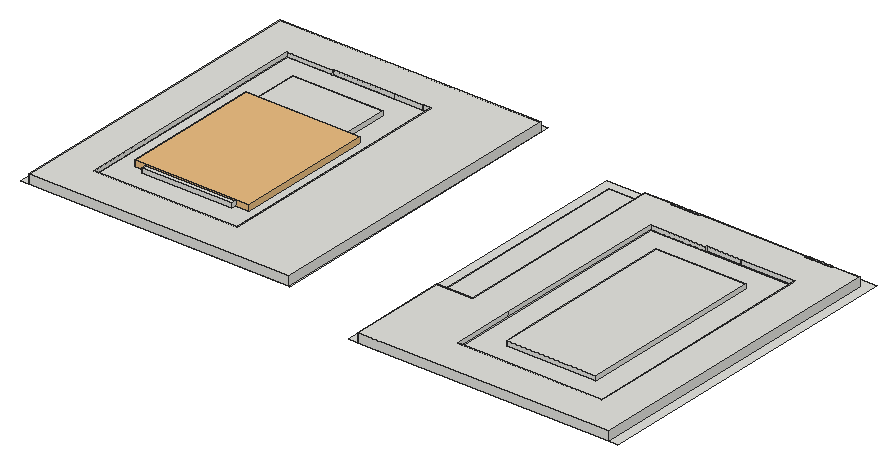
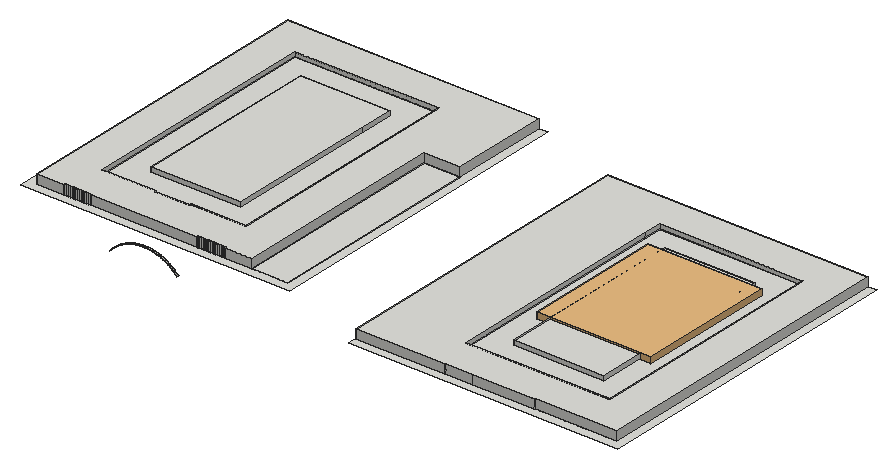
# SketchUp Ruby script. Lengths in inches.
U = 1.inch
M = Sketchup.active_model
def pt(a) = Geom::Point3d.new(a.map { |v| v * U })
def face(e, loops, mat)
  f = e.add_face(loops[0].map { |a| pt(a) })
  loops[1..].each { |l| e.add_face(l.map { |a| pt(a) }).erase! }
  f.material = f.back_material = mat if mat
  f
end
# faces: each face lists its corners as indices into pts; further lists are holes
def faces(e, pts, list, mat = nil) = list.each { |f| face(e, (f[0].is_a?(Array) ? f : [f]).map { |l| l.map { |i| pts[i] } }, mat) }
# xy, xz, yz: faces in a plane at the given z, y or x. An outline is a flat list of corners, or four numbers for a rectangle; further outlines are holes
def ring(l) = l.size == 4 ? [[l[0], l[1]], [l[2], l[1]], [l[2], l[3]], [l[0], l[3]]] : l.each_slice(2).to_a
def flat(e, list, mat, &to3) = list.each { |f| face(e, (f[0].is_a?(Array) ? f : [f]).map { |l| ring(l).map { |u, v| to3.(u, v) } }, mat) }
def xy(e, z, list, mat = nil) = flat(e, list, mat) { |x, y| [x, y, z] }
def xz(e, y, list, mat = nil) = flat(e, list, mat) { |x, z| [x, y, z] }
def yz(e, x, list, mat = nil) = flat(e, list, mat) { |y, z| [x, y, z] }
def lines(e, pts, list) = list.each { |a, b| e.add_line(pt(pts[a]), pt(pts[b])) }
# prism: a flat outline (further loops are holes) pulled along v
def prism(e, loops, v, mat = nil)
  f = face(e, loops, mat); d = Geom::Vector3d.new(v.map { |x| x * U })
  f.pushpull(f.normal.samedirection?(d) ? d.length : -d.length)
end
def box(e, o, s, mat = nil) = prism(e, [[o, [o[0] + s[0], o[1], o[2]], [o[0] + s[0], o[1] + s[1], o[2]], [o[0], o[1] + s[1], o[2]]]], [0, 0, s[2]], mat)
def at(x, y, z, deg = 0) = Geom::Transformation.translation(pt([x, y, z])) * Geom::Transformation.rotation(ORIGIN, Z_AXIS, deg.degrees)
def axes(o, x, y, z) = Geom::Transformation.new([*x, 0, *y, 0, *z, 0, *pt(o).to_a, 1])
def part(name) = M.definitions.add(name)
# library, detail: a bought-in or finely detailed component or shape, given as its bounding box
def library(name, o, s) = part(name).tap { |d| box(d.entities, o, s) }
def detail(e, o, s) = box(e.add_group.entities, o, s)
def put(e, d, t, mat = nil) = e.add_instance(d, t).tap { |i| i.material = mat if mat }
def group(e, t, mat = nil) = e.add_group.tap { |g| g.transformation = t; g.material = mat if mat }.entities
root = M.entities
M.materials.add("[Color M00]").color = [255, 255, 255]
c1 = library("ceiling fan",[0,0,0],[76.25,93.13,30.02])
c2 = part("Component\#2")
xy(c2.entities,0,[[3.27,0,4.25,0.01,5.2,0.27,6.04,0.77,6.72,1.47,7.2,2.33,7.45,3.27,7.44,4.25,7.17,5.2,6.67,6.04,5.97,6.72,5.12,7.2,4.17,7.45,3.19,7.44,2.25,7.17,1.41,6.67,0.72,5.97,0.24,5.12,0,4.17,0.01,3.19,0.27,2.25,0.77,1.41,1.47,0.72,2.33,0.24]],"[Color M00]")
xy(root,117.8,[[268.823,66.2,269.003,89.8],[268.823,90.2,269.003,113.8],[268.823,114.2,269.003,137.8],[268.823,138.2,269.003,161.8],[268.823,162.2,269.003,185.8],
  [268.823,186.2,269.003,209.8]])
xy(root,118,[[245.003,66,268.823,210],[268.823,66,269.003,210]])
xy(root,118.8,[[150,61.77,150.18,89.203],[150,89.603,150.18,118.037],[150,118.437,150.18,146.87],[150,147.27,150.18,175.703],[150,176.103,150.18,204.537],
  [150,204.937,150.18,233.37]])
xy(root,119,[[150,61.57,150.18,233.57]])
xy(root,120,[[239.003,0,245.003,0,245.003,210,413.003,210,413.003,0,419.003,0,419.003,216,239.003,216],[[245.003,0,245.003,66,269.003,66,269.003,210,287.003,210,287.003,209,288.003,209,288.003,210,288.203,210,288.203,209,289.203,209,289.203,210,289.403,210,289.403,209,290.403,209,290.403,210,290.603,210,290.603,209,291.603,209,291.603,210,291.803,210,291.803,209,292.803,209,292.803,210,293.003,210,293.003,209,294.003,209,294.003,210,294.203,210,294.203,209,295.203,209,295.203,210,295.403,210,295.403,209,296.403,209,296.403,210,296.603,210,296.603,209,297.603,209,297.603,210,297.803,210,297.803,209,298.803,209,298.803,210,299.003,210,299.003,209,300.003,209,300.003,210,300.203,210,300.203,209,301.203,209,301.203,210,301.403,210,301.403,209,302.403,209,302.403,210,302.603,210,302.603,209,303.603,209,303.603,210,303.803,210,303.803,209,304.803,209,304.803,210,305.003,210,305.003,209,306.003,209,306.003,210,377.003,210,377.003,209,378.003,209,378.003,210,378.203,210,378.203,209,379.203,209,379.203,210,379.403,210,379.403,209,380.403,209,380.403,210,380.603,210,380.603,209,381.603,209,381.603,210,381.803,210,381.803,209,382.803,209,382.803,210,383.003,210,383.003,209,384.003,209,384.003,210,384.203,210,384.203,209,385.203,209,385.203,210,385.403,210,385.403,209,386.403,209,386.403,210,386.603,210,386.603,209,387.603,209,387.603,210,387.803,210,387.803,209,388.803,209,388.803,210,389.003,210,389.003,209,390.166,209,390.166,210,390.366,210,390.366,209,391.366,209,391.366,210,391.566,210,391.566,209,392.728,209,392.728,210,392.928,210,392.928,209,393.928,209,393.928,210,394.128,210,394.128,209,395.003,209,395.003,210,413.003,210,413.003,0],[293.003,24,389.003,185],[313.331,193.1875,314.608,193.365,315.795,193.867,316.812,194.659,317.589,195.687,318.074,196.881,318.233,198.16,318.056,199.437,317.554,200.624,316.762,201.641,315.734,202.419,314.539,202.903,313.26,203.0625,311.984,202.885,310.796,202.383,309.779,201.591,309.002,200.563,308.517,199.369,308.358,198.09,308.536,196.813,309.038,195.626,309.83,194.609,310.858,193.831,312.052,193.347],[357.331,193.1875,358.608,193.365,359.795,193.867,360.812,194.659,361.589,195.687,362.074,196.881,362.233,198.16,362.056,199.437,361.554,200.624,360.762,201.641,359.734,202.419,358.539,202.903,357.26,203.0625,355.984,202.885,354.796,202.383,353.779,201.591,353.002,200.563,352.517,199.369,352.358,198.09,352.536,196.813,353.038,195.626,353.83,194.609,354.858,193.831,356.052,193.347],[281.456,7.0625,282.733,7.24,283.92,7.742,284.937,8.534,285.714,9.562,286.199,10.756,286.358,12.035,286.181,13.312,285.679,14.499,284.887,15.516,283.859,16.294,282.664,16.778,281.385,16.9375,280.109,16.76,278.921,16.258,277.904,15.466,277.127,14.438,276.642,13.244,276.483,11.965,276.661,10.688,277.163,9.501,277.955,8.484,278.983,7.706,280.177,7.222],[399.769,7.0625,401.045,7.24,402.233,7.742,403.25,8.534,404.027,9.562,404.512,10.756,404.671,12.035,404.493,13.312,403.991,14.499,403.199,15.516,402.171,16.294,400.977,16.778,399.698,16.9375,398.421,16.76,397.234,16.258,396.217,15.466,395.44,14.438,394.955,13.244,394.796,11.965,394.973,10.688,395.475,9.501,396.267,8.484,397.295,7.706,398.49,7.222],[313.331,7.0625,314.608,7.24,315.795,7.742,316.812,8.534,317.589,9.562,318.074,10.756,318.233,12.035,318.056,13.312,317.554,14.499,316.762,15.516,315.734,16.294,314.539,16.778,313.26,16.9375,311.984,16.76,310.796,16.258,309.779,15.466,309.002,14.438,308.517,13.244,308.358,11.965,308.536,10.688,309.038,9.501,309.83,8.484,310.858,7.706,312.052,7.222],[357.331,7.0625,358.608,7.24,359.795,7.742,360.812,8.534,361.589,9.562,362.074,10.756,362.233,12.035,362.056,13.312,361.554,14.499,360.762,15.516,359.734,16.294,358.539,16.778,357.26,16.9375,355.984,16.76,354.796,16.258,353.779,15.466,353.002,14.438,352.517,13.244,352.358,11.965,352.536,10.688,353.038,9.501,353.83,8.484,354.858,7.706,356.052,7.222],[281.456,89.875,282.733,90.053,283.92,90.554,284.937,91.346,285.714,92.374,286.199,93.569,286.358,94.848,286.181,96.125,285.679,97.312,284.887,98.329,283.859,99.106,282.664,99.591,281.385,99.75,280.109,99.572,278.921,99.071,277.904,98.279,277.127,97.251,276.642,96.056,276.483,94.777,276.661,93.5,277.163,92.313,277.955,91.296,278.983,90.519,280.177,90.034],[399.769,89.875,401.045,90.053,402.233,90.554,403.25,91.346,404.027,92.374,404.512,93.569,404.671,94.848,404.493,96.125,403.991,97.312,403.199,98.329,402.171,99.106,400.977,99.591,399.698,99.75,398.421,99.572,397.234,99.071,396.217,98.279,395.44,97.251,394.955,96.056,394.796,94.777,394.973,93.5,395.475,92.313,396.267,91.296,397.295,90.519,398.49,90.034],[399.769,53.6875,401.045,53.865,402.233,54.367,403.25,55.159,404.027,56.187,404.512,57.381,404.671,58.66,404.493,59.937,403.991,61.124,403.199,62.141,402.171,62.919,400.977,63.403,399.698,63.5625,398.421,63.385,397.234,62.883,396.217,62.091,395.44,61.063,394.955,59.869,394.796,58.59,394.973,57.313,395.475,56.126,396.267,55.109,397.295,54.331,398.49,53.847],[281.456,53.6875,282.733,53.865,283.92,54.367,284.937,55.159,285.714,56.187,286.199,57.381,286.358,58.66,286.181,59.937,285.679,61.124,284.887,62.141,283.859,62.919,282.664,63.403,281.385,63.5625,280.109,63.385,278.921,62.883,277.904,62.091,277.127,61.063,276.642,59.869,276.483,58.59,276.661,57.313,277.163,56.126,277.955,55.109,278.983,54.331,280.177,53.847],[281.456,137.125,282.733,137.303,283.92,137.804,284.937,138.596,285.714,139.624,286.199,140.819,286.358,142.098,286.181,143.375,285.679,144.562,284.887,145.579,283.859,146.356,282.664,146.841,281.385,147,280.109,146.822,278.921,146.321,277.904,145.529,277.127,144.501,276.642,143.306,276.483,142.027,276.661,140.75,277.163,139.563,277.955,138.546,278.983,137.769,280.177,137.284],[399.769,137.125,401.045,137.303,402.233,137.804,403.25,138.596,404.027,139.624,404.512,140.819,404.671,142.098,404.493,143.375,403.991,144.562,403.199,145.579,402.171,146.356,400.977,146.841,399.698,147,398.421,146.822,397.234,146.321,396.217,145.529,395.44,144.501,394.955,143.306,394.796,142.027,394.973,140.75,395.475,139.563,396.267,138.546,397.295,137.769,398.49,137.284],[281.456,190.125,282.733,190.303,283.92,190.804,284.937,191.596,285.714,192.624,286.199,193.819,286.358,195.098,286.181,196.375,285.679,197.562,284.887,198.579,283.859,199.356,282.664,199.841,281.385,200,280.109,199.822,278.921,199.321,277.904,198.529,277.127,197.501,276.642,196.306,276.483,195.027,276.661,193.75,277.163,192.563,277.955,191.546,278.983,190.769,280.177,190.284],[399.769,190.125,401.045,190.303,402.233,190.804,403.25,191.596,404.027,192.624,404.512,193.819,404.671,195.098,404.493,196.375,403.991,197.562,403.199,198.579,402.171,199.356,400.977,199.841,399.698,200,398.421,199.822,397.234,199.321,396.217,198.529,395.44,197.501,394.955,196.306,394.796,195.027,394.973,193.75,395.475,192.563,396.267,191.546,397.295,190.769,398.49,190.284]],[281.456,7.0625,280.177,7.222,278.983,7.706,277.955,8.484,277.163,9.501,276.661,10.688,276.483,11.965,276.642,13.244,277.127,14.438,277.904,15.466,278.921,16.258,280.109,16.76,281.385,16.9375,282.664,16.778,283.859,16.294,284.887,15.516,285.679,14.499,286.181,13.312,286.358,12.035,286.199,10.756,285.714,9.562,284.937,8.534,283.92,7.742,282.733,7.24],[313.331,7.0625,312.052,7.222,310.858,7.706,309.83,8.484,309.038,9.501,308.536,10.688,308.358,11.965,308.517,13.244,309.002,14.438,309.779,15.466,310.796,16.258,311.984,16.76,313.26,16.9375,314.539,16.778,315.734,16.294,316.762,15.516,317.554,14.499,318.056,13.312,318.233,12.035,318.074,10.756,317.589,9.562,316.812,8.534,315.795,7.742,314.608,7.24],[357.331,7.0625,356.052,7.222,354.858,7.706,353.83,8.484,353.038,9.501,352.536,10.688,352.358,11.965,352.517,13.244,353.002,14.438,353.779,15.466,354.796,16.258,355.984,16.76,357.26,16.9375,358.539,16.778,359.734,16.294,360.762,15.516,361.554,14.499,362.056,13.312,362.233,12.035,362.074,10.756,361.589,9.562,360.812,8.534,359.795,7.742,358.608,7.24],
  [399.769,7.0625,398.49,7.222,397.295,7.706,396.267,8.484,395.475,9.501,394.973,10.688,394.796,11.965,394.955,13.244,395.44,14.438,396.217,15.466,397.234,16.258,398.421,16.76,399.698,16.9375,400.977,16.778,402.171,16.294,403.199,15.516,403.991,14.499,404.493,13.312,404.671,12.035,404.512,10.756,404.027,9.562,403.25,8.534,402.233,7.742,401.045,7.24],[0,24.57,0,240.57,180,240.57,180,24.57,179.625,24.57,179.625,234.57,5.625,234.57,5.625,24.57],[5.625,24.57,6,234.57],[[6,24.57,6,234.57,150,234.57,150,60.57,174,60.57,174,24.57],[29.625,48.57,125.625,210.57]],[174,24.57,179.625,234.57],
  [281.456,53.6875,280.177,53.847,278.983,54.331,277.955,55.109,277.163,56.126,276.661,57.313,276.483,58.59,276.642,59.869,277.127,61.063,277.904,62.091,278.921,62.883,280.109,63.385,281.385,63.5625,282.664,63.403,283.859,62.919,284.887,62.141,285.679,61.124,286.181,59.937,286.358,58.66,286.199,57.381,285.714,56.187,284.937,55.159,283.92,54.367,282.733,53.865],[399.769,53.6875,398.49,53.847,397.295,54.331,396.267,55.109,395.475,56.126,394.973,57.313,394.796,58.59,394.955,59.869,395.44,61.063,396.217,62.091,397.234,62.883,398.421,63.385,399.698,63.5625,400.977,63.403,402.171,62.919,403.199,62.141,403.991,61.124,404.493,59.937,404.671,58.66,404.512,57.381,404.027,56.187,403.25,55.159,402.233,54.367,401.045,53.865],[150,60.57,174,234.57],[245.003,66,269.003,210],[281.456,89.875,280.177,90.034,278.983,90.519,277.955,91.296,277.163,92.313,276.661,93.5,276.483,94.777,276.642,96.056,277.127,97.251,277.904,98.279,278.921,99.071,280.109,99.572,281.385,99.75,282.664,99.591,283.859,99.106,284.887,98.329,285.679,97.312,286.181,96.125,286.358,94.848,286.199,93.569,285.714,92.374,284.937,91.346,283.92,90.554,282.733,90.053],
  [399.769,89.875,398.49,90.034,397.295,90.519,396.267,91.296,395.475,92.313,394.973,93.5,394.796,94.777,394.955,96.056,395.44,97.251,396.217,98.279,397.234,99.071,398.421,99.572,399.698,99.75,400.977,99.591,402.171,99.106,403.199,98.329,403.991,97.312,404.493,96.125,404.671,94.848,404.512,93.569,404.027,92.374,403.25,91.346,402.233,90.554,401.045,90.053],[281.456,137.125,280.177,137.284,278.983,137.769,277.955,138.546,277.163,139.563,276.661,140.75,276.483,142.027,276.642,143.306,277.127,144.501,277.904,145.529,278.921,146.321,280.109,146.822,281.385,147,282.664,146.841,283.859,146.356,284.887,145.579,285.679,144.562,286.181,143.375,286.358,142.098,286.199,140.819,285.714,139.624,284.937,138.596,283.92,137.804,282.733,137.303],[399.769,137.125,398.49,137.284,397.295,137.769,396.267,138.546,395.475,139.563,394.973,140.75,394.796,142.027,394.955,143.306,395.44,144.501,396.217,145.529,397.234,146.321,398.421,146.822,399.698,147,400.977,146.841,402.171,146.356,403.199,145.579,403.991,144.562,404.493,143.375,404.671,142.098,404.512,140.819,404.027,139.624,403.25,138.596,402.233,137.804,401.045,137.303],[281.456,190.125,280.177,190.284,278.983,190.769,277.955,191.546,277.163,192.563,276.661,193.75,276.483,195.027,276.642,196.306,277.127,197.501,277.904,198.529,278.921,199.321,280.109,199.822,281.385,200,282.664,199.841,283.859,199.356,284.887,198.579,285.679,197.562,286.181,196.375,286.358,195.098,286.199,193.819,285.714,192.624,284.937,191.596,283.92,190.804,282.733,190.303],[399.769,190.125,398.49,190.284,397.295,190.769,396.267,191.546,395.475,192.563,394.973,193.75,394.796,195.027,394.955,196.306,395.44,197.501,396.217,198.529,397.234,199.321,398.421,199.822,399.698,200,400.977,199.841,402.171,199.356,403.199,198.579,403.991,197.562,404.493,196.375,404.671,195.098,404.512,193.819,404.027,192.624,403.25,191.596,402.233,190.804,401.045,190.303],
  [313.331,193.1875,312.052,193.347,310.858,193.831,309.83,194.609,309.038,195.626,308.536,196.813,308.358,198.09,308.517,199.369,309.002,200.563,309.779,201.591,310.796,202.383,311.984,202.885,313.26,203.0625,314.539,202.903,315.734,202.419,316.762,201.641,317.554,200.624,318.056,199.437,318.233,198.16,318.074,196.881,317.589,195.687,316.812,194.659,315.795,193.867,314.608,193.365],[357.331,193.1875,356.052,193.347,354.858,193.831,353.83,194.609,353.038,195.626,352.536,196.813,352.358,198.09,352.517,199.369,353.002,200.563,353.779,201.591,354.796,202.383,355.984,202.885,357.26,203.0625,358.539,202.903,359.734,202.419,360.762,201.641,361.554,200.624,362.056,199.437,362.233,198.16,362.074,196.881,361.589,195.687,360.812,194.659,359.795,193.867,358.608,193.365],[287.003,209,288.003,210],[288.203,209,289.203,210],[289.403,209,290.403,210],
  [290.603,209,291.603,210],[291.803,209,292.803,210],[293.003,209,294.003,210],[294.203,209,295.203,210],[295.403,209,296.403,210],
  [296.603,209,297.603,210],[297.803,209,298.803,210],[299.003,209,300.003,210],[300.203,209,301.203,210],[301.403,209,302.403,210],
  [302.603,209,303.603,210],[303.803,209,304.803,210],[305.003,209,306.003,210],[377.003,209,378.003,210],[378.203,209,379.203,210],
  [379.403,209,380.403,210],[380.603,209,381.603,210],[381.803,209,382.803,210],[383.003,209,384.003,210],[384.203,209,385.203,210],
  [385.403,209,386.403,210],[386.603,209,387.603,210],[387.803,209,388.803,210],[389.003,209,390.166,210],[390.366,209,391.366,210],
  [391.566,209,392.728,210],[392.928,209,393.928,210],[394.128,209,395.003,210]])
xy(root,123,[[[293.003,24,389.003,185],[311.003,42,371.003,167]],[[29.625,48.57,125.625,210.57],[47.625,66.57,107.625,192.57]],[330.003,185,353.003,186]])
xy(root,126,[[[245.003,0,413.003,0,413.003,210,395.003,210,395.003,209,394.128,209,394.128,210,393.928,210,393.928,209,392.928,209,392.928,210,392.728,210,392.728,209,391.566,209,391.566,210,391.366,210,391.366,209,390.366,209,390.366,210,390.166,210,390.166,209,389.003,209,389.003,210,388.803,210,388.803,209,387.803,209,387.803,210,387.603,210,387.603,209,386.603,209,386.603,210,386.403,210,386.403,209,385.403,209,385.403,210,385.203,210,385.203,209,384.203,209,384.203,210,384.003,210,384.003,209,383.003,209,383.003,210,382.803,210,382.803,209,381.803,209,381.803,210,381.603,210,381.603,209,380.603,209,380.603,210,380.403,210,380.403,209,379.403,209,379.403,210,379.203,210,379.203,209,378.203,209,378.203,210,378.003,210,378.003,209,377.003,209,377.003,210,306.003,210,306.003,209,305.003,209,305.003,210,304.803,210,304.803,209,303.803,209,303.803,210,303.603,210,303.603,209,302.603,209,302.603,210,302.403,210,302.403,209,301.403,209,301.403,210,301.203,210,301.203,209,300.203,209,300.203,210,300.003,210,300.003,209,299.003,209,299.003,210,298.803,210,298.803,209,297.803,209,297.803,210,297.603,210,297.603,209,296.603,209,296.603,210,296.403,210,296.403,209,295.403,209,295.403,210,295.203,210,295.203,209,294.203,209,294.203,210,294.003,210,294.003,209,293.003,209,293.003,210,292.803,210,292.803,209,291.803,209,291.803,210,291.603,210,291.603,209,290.603,209,290.603,210,290.403,210,290.403,209,289.403,209,289.403,210,289.203,210,289.203,209,288.203,209,288.203,210,288.003,210,288.003,209,287.003,209,287.003,210,269.003,210,269.003,66,245.003,66],[293.003,24,293.003,185,330.003,185,330.003,186,353.003,186,353.003,185,389.003,185,389.003,24]],[[5.625,24.57,179.625,234.57],[29.625,48.57,125.625,210.57]],[311.003,42,371.003,167],[47.625,66.57,107.625,192.57]])
xz(root,0,[[245.003,120,413.003,126]])
xz(root,24,[[293.003,120,389.003,123],[293.003,123,389.003,126]])
xz(root,24.57,[[5.625,120,179.625,126]])
xz(root,42,[[311.003,123,371.003,126]])
xz(root,48.57,[[29.625,120,125.625,123],[29.625,123,125.625,126]])
xz(root,66,[[245.003,118,269.003,120],[245.003,120,269.003,126]])
xz(root,66.57,[[47.625,123,107.625,126]])
xz(root,167,[[311.003,123,371.003,126]])
xz(root,185,[[293.003,120,389.003,123],[293.003,123,330.003,126],[353.003,123,389.003,126]])
xz(root,186,[[330.003,123,353.003,126]])
xz(root,192.57,[[47.625,123,107.625,126]])
xz(root,209,[[287.003,120,288.003,126],[288.203,120,289.203,126],[289.403,120,290.403,126],[290.603,120,291.603,126],[291.803,120,292.803,126],
  [293.003,120,294.003,126],[294.203,120,295.203,126],[295.403,120,296.403,126],[296.603,120,297.603,126],[297.803,120,298.803,126],
  [299.003,120,300.003,126],[300.203,120,301.203,126],[301.403,120,302.403,126],[302.603,120,303.603,126],[303.803,120,304.803,126],
  [305.003,120,306.003,126],[377.003,120,378.003,126],[378.203,120,379.203,126],[379.403,120,380.403,126],[380.603,120,381.603,126],
  [381.803,120,382.803,126],[383.003,120,384.003,126],[384.203,120,385.203,126],[385.403,120,386.403,126],[386.603,120,387.603,126],
  [387.803,120,388.803,126],[389.003,120,390.166,126],[390.366,120,391.366,126],[391.566,120,392.728,126],[392.928,120,393.928,126],
  [394.128,120,395.003,126]])
xz(root,210,[[245.003,118,269.003,120],[269.003,120,287.003,126],[288.003,120,288.203,126],[289.203,120,289.403,126],[290.403,120,290.603,126],
  [291.603,120,291.803,126],[292.803,120,293.003,126],[294.003,120,294.203,126],[295.203,120,295.403,126],[296.403,120,296.603,126],
  [297.603,120,297.803,126],[298.803,120,299.003,126],[300.003,120,300.203,126],[301.203,120,301.403,126],[302.403,120,302.603,126],
  [303.603,120,303.803,126],[304.803,120,305.003,126],[306.003,120,377.003,126],[378.003,120,378.203,126],[379.203,120,379.403,126],
  [380.403,120,380.603,126],[381.603,120,381.803,126],[382.803,120,383.003,126],[384.003,120,384.203,126],[385.203,120,385.403,126],
  [386.403,120,386.603,126],[387.603,120,387.803,126],[388.803,120,389.003,126],[390.166,120,390.366,126],[391.366,120,391.566,126],
  [392.728,120,392.928,126],[393.928,120,394.128,126],[395.003,120,413.003,126]])
xz(root,210.57,[[29.625,120,125.625,123],[29.625,123,59.625,126],[59.625,123,60.625,126],[60.625,123,101.625,126],[101.625,123,119.625,126],
  [119.625,123,120.625,126],[120.625,123,125.625,126]])
xz(root,234.57,[[5.625,120,59.625,126],[59.625,120,60.625,126],[60.625,120,101.625,126],[101.625,120,119.625,126],[119.625,120,120.625,126],
  [120.625,120,179.625,126]])
yz(root,5.625,[[24.57,120,234.57,126]])
yz(root,29.625,[[48.57,120,210.57,123],[48.57,123,210.57,126]])
yz(root,47.625,[[66.57,123,192.57,126]])
yz(root,107.625,[[66.57,123,192.57,126]])
yz(root,125.625,[[48.57,120,60.57,123],[60.57,120,210.57,123],[48.57,123,60.57,126],[60.57,123,210.57,126]])
yz(root,179.625,[[24.57,120,234.57,126]])
yz(root,245.003,[[66,118,210,120],[0,120,66,126]])
yz(root,269.003,[[66,118,210,120],[66,120,210,126]])
yz(root,287.003,[[209,120,210,126]])
yz(root,288.003,[[209,120,210,126]])
yz(root,288.203,[[209,120,210,126]])
yz(root,289.203,[[209,120,210,126]])
yz(root,289.403,[[209,120,210,126]])
yz(root,290.403,[[209,120,210,126]])
yz(root,290.603,[[209,120,210,126]])
yz(root,291.603,[[209,120,210,126]])
yz(root,291.803,[[209,120,210,126]])
yz(root,292.803,[[209,120,210,126]])
yz(root,293.003,[[24,120,66,123],[66,120,185,123],[209,120,210,126],[24,123,66,126],[66,123,185,126]])
yz(root,294.003,[[209,120,210,126]])
yz(root,294.203,[[209,120,210,126]])
yz(root,295.203,[[209,120,210,126]])
yz(root,295.403,[[209,120,210,126]])
yz(root,296.403,[[209,120,210,126]])
yz(root,296.603,[[209,120,210,126]])
yz(root,297.603,[[209,120,210,126]])
yz(root,297.803,[[209,120,210,126]])
yz(root,298.803,[[209,120,210,126]])
yz(root,299.003,[[209,120,210,126]])
yz(root,300.003,[[209,120,210,126]])
yz(root,300.203,[[209,120,210,126]])
yz(root,301.203,[[209,120,210,126]])
yz(root,301.403,[[209,120,210,126]])
yz(root,302.403,[[209,120,210,126]])
yz(root,302.603,[[209,120,210,126]])
yz(root,303.603,[[209,120,210,126]])
yz(root,303.803,[[209,120,210,126]])
yz(root,304.803,[[209,120,210,126]])
yz(root,305.003,[[209,120,210,126]])
yz(root,306.003,[[209,120,210,126]])
yz(root,311.003,[[42,123,66,126],[66,123,167,126]])
yz(root,330.003,[[185,123,186,126]])
yz(root,353.003,[[185,123,186,126]])
yz(root,371.003,[[42,123,167,126]])
yz(root,377.003,[[209,120,210,126]])
yz(root,378.003,[[209,120,210,126]])
yz(root,378.203,[[209,120,210,126]])
yz(root,379.203,[[209,120,210,126]])
yz(root,379.403,[[209,120,210,126]])
yz(root,380.403,[[209,120,210,126]])
yz(root,380.603,[[209,120,210,126]])
yz(root,381.603,[[209,120,210,126]])
yz(root,381.803,[[209,120,210,126]])
yz(root,382.803,[[209,120,210,126]])
yz(root,383.003,[[209,120,210,126]])
yz(root,384.003,[[209,120,210,126]])
yz(root,384.203,[[209,120,210,126]])
yz(root,385.203,[[209,120,210,126]])
yz(root,385.403,[[209,120,210,126]])
yz(root,386.403,[[209,120,210,126]])
yz(root,386.603,[[209,120,210,126]])
yz(root,387.603,[[209,120,210,126]])
yz(root,387.803,[[209,120,210,126]])
yz(root,388.803,[[209,120,210,126]])
yz(root,389.003,[[24,120,185,123],[209,120,210,126],[24,123,185,126]])
yz(root,390.166,[[209,120,210,126]])
yz(root,390.366,[[209,120,210,126]])
yz(root,391.366,[[209,120,210,126]])
yz(root,391.566,[[209,120,210,126]])
yz(root,392.728,[[209,120,210,126]])
yz(root,392.928,[[209,120,210,126]])
yz(root,393.928,[[209,120,210,126]])
yz(root,394.128,[[209,120,210,126]])
yz(root,395.003,[[209,120,210,126]])
yz(root,413.003,[[0,120,210,126]])
p = [[363.909,210,97.228],[363.398,210,97.811],[363.398,209,97.811],[363.909,209,97.228],[319.394,210,97.811],[318.953,210,97.307],
  [318.953,209,97.307],[319.394,209,97.811],[319.921,210,98.38],[319.921,209,98.38],[363.353,210,97.86],[363.353,209,97.86],
  [363.153,210,98.076],[362.872,210,98.38],[362.872,209,98.38],[363.153,209,98.076],[319.953,210,98.413],[319.953,209,98.413],
  [362.331,210,98.935],[362.331,209,98.935],[320.461,210,98.935],[320.153,210,98.619],[320.153,209,98.619],[320.461,209,98.935],
  [321.017,210,99.476],[321.017,209,99.476],[362.153,210,99.109],[362.153,209,99.109],[361.953,210,99.304],[361.776,210,99.476],
  [361.776,209,99.476],[361.953,209,99.304],[321.153,210,99.602],[321.153,209,99.602],[361.207,210,100.002],[361.207,209,100.002],
  [321.586,210,100.002],[321.353,210,99.787],[321.353,209,99.787],[321.586,209,100.002],[322.168,210,100.513],[322.168,209,100.513],
  [360.953,210,100.225],[360.953,209,100.225],[360.753,210,100.4],[360.624,210,100.513],[360.624,209,100.513],[360.753,209,100.4],
  [322.353,210,100.667],[322.353,209,100.667],[360.028,210,101.009],[360.028,209,101.009],[322.764,210,101.009],[322.553,210,100.833],
  [322.553,209,100.833],[322.764,209,101.009],[323.373,210,101.489],[323.373,209,101.489],[359.753,210,101.226],[359.753,209,101.226],
  [359.553,210,101.383],[359.42,210,101.489],[359.42,209,101.489],[359.553,209,101.383],[323.553,210,101.623],[323.553,209,101.623],
  [358.799,210,101.952],[358.799,209,101.952],[323.994,210,101.952],[323.753,210,101.772],[323.753,209,101.772],[323.994,209,101.952],
  [324.627,210,102.4],[324.627,209,102.4],[358.553,210,102.126],[358.553,209,102.126],[358.353,210,102.267],[358.166,210,102.4],
  [358.166,209,102.4],[358.353,209,102.267],[324.753,210,102.484],[324.753,209,102.484],[357.521,210,102.83],[357.521,209,102.83],
  [325.271,210,102.83],[324.953,210,102.617],[324.953,209,102.617],[325.271,209,102.83],[325.927,210,103.244],[325.927,209,103.244],
  [357.353,210,102.936],[357.353,209,102.936],[357.153,210,103.0625],[356.866,210,103.244],[356.866,209,103.244],[357.153,209,103.0625],
  [325.953,210,103.259],[325.953,209,103.259],[356.2,210,103.64],[356.2,209,103.64],[326.593,210,103.64],[326.153,210,103.378],
  [326.153,209,103.378],[326.593,209,103.64],[327.153,210,103.954],[327.153,209,103.954],[356.153,210,103.666],[356.153,209,103.666],
  [355.953,210,103.778],[355.523,210,104.019],[355.523,209,104.019],[355.953,209,103.778],[354.953,210,104.319],[354.953,209,104.319],
  [327.955,210,104.38],[327.353,210,104.063],[327.353,209,104.063],[327.955,209,104.38],[328.353,210,104.576],[328.353,209,104.576],
  [354.753,210,104.421],[354.142,210,104.723],[354.142,209,104.723],[354.753,209,104.421],[328.65,210,104.723],[328.553,210,104.675],
  [328.553,209,104.675],[328.65,209,104.723],[329.354,210,105.047],[329.354,209,105.047],[353.753,210,104.902],[353.753,209,104.902],
  [329.553,210,105.132],[329.553,209,105.132],[353.439,210,105.047],[352.726,210,105.353],[352.726,209,105.353],[353.439,209,105.047],
  [353.553,210,104.994],[353.553,209,104.994],[330.066,210,105.353],[329.753,210,105.218],[329.753,209,105.218],[330.066,209,105.353],
  [330.753,210,105.627],[330.753,209,105.627],[352.553,210,105.422],[352.553,209,105.422],[352.353,210,105.502],[352.006,210,105.64],
  [352.006,209,105.64],[352.353,209,105.502],[351.353,210,105.881],[351.353,209,105.881],[331.514,210,105.908],[330.953,210,105.702],
  [330.953,209,105.702],[331.514,209,105.908],[331.953,210,106.058],[331.953,209,106.058],[351.153,210,105.951],[350.545,210,106.158],
  [350.545,209,106.158],[351.153,209,105.951],[332.247,210,106.158],[332.153,210,106.126],[332.153,209,106.126],[332.247,209,106.158],
  [332.988,210,106.387],[332.988,209,106.387],[350.153,210,106.279],[350.153,209,106.279],[349.953,210,106.342],[349.805,210,106.387],
  [349.805,209,106.387],[349.953,209,106.342],[333.153,210,106.434],[333.153,209,106.434],[349.059,210,106.598],[349.059,209,106.598],
  [333.734,210,106.598],[333.353,210,106.49],[333.353,209,106.49],[333.734,209,106.598],[334.353,210,106.755],[334.353,209,106.755],
  [348.953,210,106.625],[348.953,209,106.625],[348.753,210,106.676],[348.308,210,106.789],[348.308,209,106.789],[348.753,209,106.676],
  [335.241,210,106.96],[334.553,210,106.804],[334.553,209,106.804],[335.241,209,106.96],[347.753,210,106.914],[347.753,209,106.914],
  [335.553,210,107.022],[335.553,209,107.022],[347.552,210,106.96],[346.792,210,107.111],[346.792,209,107.111],[347.552,209,106.96],
  [347.553,210,106.959],[347.553,209,106.959],[336.001,210,107.111],[335.753,210,107.062],[335.753,209,107.062],[336.001,209,107.111],
  [336.753,210,107.24],[336.753,209,107.24],[346.553,210,107.152],[346.553,209,107.152],[346.028,210,107.242],[345.353,210,107.34],
  [345.353,209,107.34],[346.028,209,107.242],[346.353,210,107.186],[346.353,209,107.186],[337.532,210,107.353],[336.953,210,107.269],
  [336.953,209,107.269],[337.532,209,107.353],[337.953,210,107.403],[337.953,209,107.403],[338.302,210,107.444],[338.153,210,107.427],
  [338.153,209,107.427],[338.302,209,107.444],[339.073,210,107.515],[339.073,209,107.515],[344.491,210,107.444],[344.153,210,107.476],
  [344.153,209,107.476],[344.491,209,107.444],[345.153,210,107.366],[345.153,209,107.366],[339.153,210,107.521],[339.153,209,107.521],
  [339.847,210,107.566],[339.353,210,107.534],[339.353,209,107.534],[339.847,209,107.566],[343.719,210,107.515],[342.953,210,107.566],
  [342.953,209,107.566],[343.719,209,107.515],[343.953,210,107.494],[343.953,209,107.494],[340.353,210,107.586],[340.353,209,107.586],
  [340.621,210,107.596],[340.553,210,107.594],[340.553,209,107.594],[340.621,209,107.596],[341.396,210,107.607],[341.396,209,107.607],
  [341.553,210,107.605],[341.553,209,107.605],[342.171,210,107.596],[341.753,210,107.602],[341.753,209,107.602],[342.171,209,107.596],
  [342.753,210,107.574],[342.753,209,107.574],[413.36,-878.15,518.819],[413.358,-878.15,518.819],[413.358,-878.15,517.783],[413.36,-878.15,517.783],
  [580.513,-265.993,540.318],[580.515,-265.994,540.318],[580.515,-265.994,541.354],[580.513,-265.993,541.354]]
faces(root,p,[[0,1,2,3],[4,5,6,7],[8,4,7,9],[1,10,11,2],[12,13,14,15],[16,8,9,17],[13,18,19,14],[20,21,22,23],
  [24,20,23,25],[18,26,27,19],[28,29,30,31],[32,24,25,33],[29,34,35,30],[36,37,38,39],[40,36,39,41],[34,42,43,35],
  [44,45,46,47],[48,40,41,49],[45,50,51,46],[52,53,54,55],[56,52,55,57],[50,58,59,51],[60,61,62,63],[64,56,57,65],
  [61,66,67,62],[68,69,70,71],[72,68,71,73],[66,74,75,67],[76,77,78,79],[80,72,73,81],[77,82,83,78],[84,85,86,87],
  [88,84,87,89],[82,90,91,83],[92,93,94,95],[96,88,89,97],[93,98,99,94],[100,101,102,103],[104,100,103,105],[98,106,107,99],
  [108,109,110,111],[109,112,113,110],[114,115,116,117],[118,114,117,119],[120,121,122,123],[124,125,126,127],[128,124,127,129],[121,130,131,122],
  [132,128,129,133],[134,135,136,137],[138,134,137,139],[140,141,142,143],[144,140,143,145],[135,146,147,136],[148,149,150,151],[149,152,153,150],
  [154,155,156,157],[158,154,157,159],[160,161,162,163],[164,165,166,167],[168,164,167,169],[161,170,171,162],[172,173,174,175],[176,168,169,177],
  [173,178,179,174],[180,181,182,183],[184,180,183,185],[178,186,187,179],[188,189,190,191],[192,193,194,195],[189,196,197,190],[198,192,195,199],
  [200,201,202,203],[204,200,203,205],[206,207,208,209],[210,206,209,211],[201,212,213,202],[214,215,216,217],[218,214,217,219],[220,221,222,223],
  [224,220,223,225],[226,227,228,229],[230,226,229,231],[232,233,234,235],[236,232,235,237],[238,230,231,239],[240,241,242,243],[244,245,246,247],
  [248,244,247,249],[250,240,243,251],[252,253,254,255],[256,252,255,257],[258,256,257,259],[260,261,262,263],[264,260,263,265]])
lines(root,p,[[266,267],[268,269],[270,271],[272,273]])
put(root,c1,axes([40.16,69.79,103.34],[1,0,0],[0,1,0],[0,0,0.78]))
put(root,c2,axes([137.86,105.63,120],[-1,0,0],[0,1,0],[0,0,-1]),"[Color M00]")
put(root,c2,axes([137.86,83.88,120],[-1,0,0],[0,1,0],[0,0,-1]),"[Color M00]")
put(root,c2,axes([137.86,60.38,120],[-1,0,0],[0,1,0],[0,0,-1]),"[Color M00]")
put(root,c2,axes([137.86,134.07,120],[-1,0,0],[0,1,0],[0,0,-1]),"[Color M00]")
put(root,c2,axes([21.92,173.51,120],[-1,0,0],[0,1,0],[0,0,-1]),"[Color M00]")
put(root,c2,axes([79.67,34.94,120],[-1,0,0],[0,1,0],[0,0,-1]),"[Color M00]")
put(root,c2,axes([21.92,83.88,120],[-1,0,0],[0,1,0],[0,0,-1]),"[Color M00]")
put(root,c2,axes([21.92,60.38,120],[-1,0,0],[0,1,0],[0,0,-1]),"[Color M00]")
put(root,c2,axes([137.86,217.94,120],[-1,0,0],[0,1,0],[0,0,-1]),"[Color M00]")
put(root,c2,axes([137.86,173.51,120],[-1,0,0],[0,1,0],[0,0,-1]),"[Color M00]")
put(root,c2,axes([21.92,134.07,120],[-1,0,0],[0,1,0],[0,0,-1]),"[Color M00]")
put(root,c2,axes([79.67,217.94,120],[-1,0,0],[0,1,0],[0,0,-1]),"[Color M00]")
put(root,c2,axes([21.92,34.94,120],[-1,0,0],[0,1,0],[0,0,-1]),"[Color M00]")
put(root,c2,axes([137.86,34.94,120],[-1,0,0],[0,1,0],[0,0,-1]),"[Color M00]")
put(root,c2,axes([21.92,217.94,120],[-1,0,0],[0,1,0],[0,0,-1]),"[Color M00]")
put(root,c2,axes([21.92,105.63,120],[-1,0,0],[0,1,0],[0,0,-1]),"[Color M00]")
